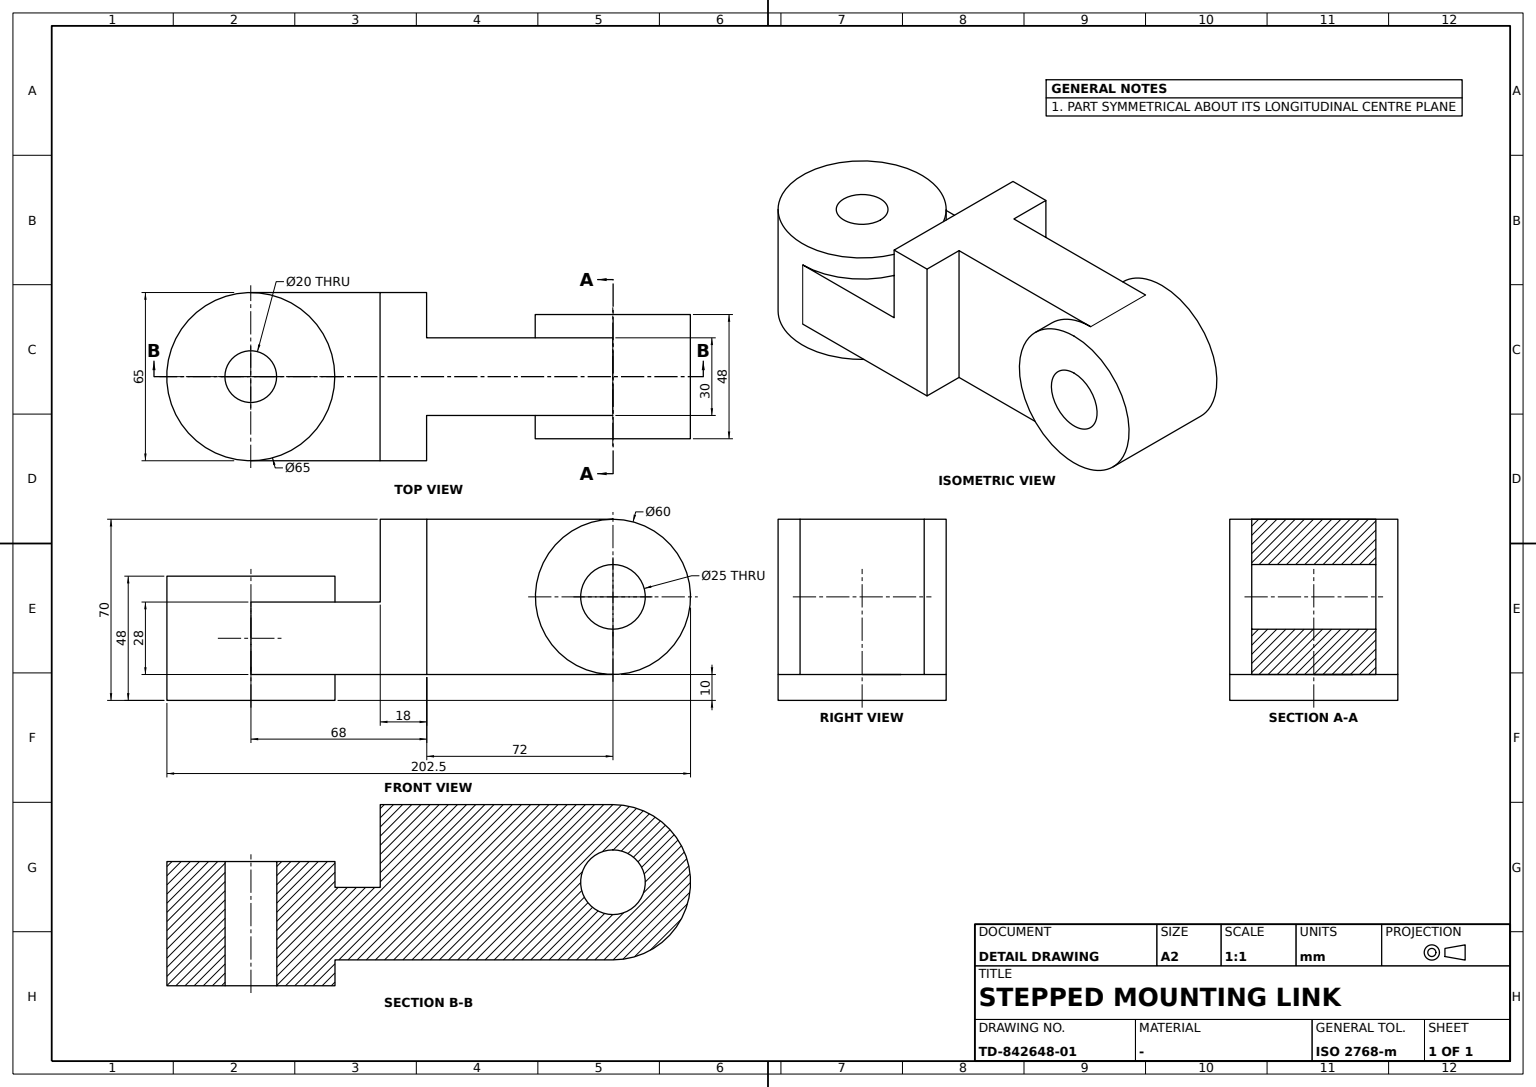
ISO-10303-21;
HEADER;
FILE_DESCRIPTION((''),'2;1');
FILE_NAME('','',(''),(''),'','','');
FILE_SCHEMA(('AUTOMOTIVE_DESIGN'));
ENDSEC;
DATA;
#1=APPLICATION_CONTEXT('');
#2=PRODUCT_CONTEXT('',#1,'mechanical');
#3=PRODUCT('','','',(#2));
#4=PRODUCT_DEFINITION_FORMATION('','',#3);
#5=PRODUCT_DEFINITION_CONTEXT('',#1,'design');
#6=PRODUCT_DEFINITION('','',#4,#5);
#7=PRODUCT_DEFINITION_SHAPE('','',#6);
#8=(LENGTH_UNIT()NAMED_UNIT(*)SI_UNIT(.MILLI.,.METRE.));
#9=(NAMED_UNIT(*)PLANE_ANGLE_UNIT()SI_UNIT($,.RADIAN.));
#10=(NAMED_UNIT(*)SI_UNIT($,.STERADIAN.)SOLID_ANGLE_UNIT());
#11=UNCERTAINTY_MEASURE_WITH_UNIT(LENGTH_MEASURE(0.005),#8,'distance_accuracy_value','');
#12=(GEOMETRIC_REPRESENTATION_CONTEXT(3)GLOBAL_UNCERTAINTY_ASSIGNED_CONTEXT((#11))GLOBAL_UNIT_ASSIGNED_CONTEXT((#8,#9,#10))REPRESENTATION_CONTEXT('',''));
#13=CARTESIAN_POINT('',(34.,-15.,0.));
#14=VERTEX_POINT('',#13);
#15=CARTESIAN_POINT('',(34.,-32.5,0.));
#16=VERTEX_POINT('',#15);
#17=CARTESIAN_POINT('',(34.,0.,0.));
#18=DIRECTION('',(0.,-1.,0.));
#19=VECTOR('',#18,1000.);
#20=LINE('',#17,#19);
#21=EDGE_CURVE('',#14,#16,#20,.T.);
#22=ORIENTED_EDGE('',*,*,#21,.F.);
#23=CARTESIAN_POINT('',(34.,-15.,60.));
#24=VERTEX_POINT('',#23);
#25=DIRECTION('',(0.,0.,-1.));
#26=VECTOR('',#25,1000.);
#27=LINE('',#13,#26);
#28=EDGE_CURVE('',#24,#14,#27,.T.);
#29=ORIENTED_EDGE('',*,*,#28,.F.);
#30=CARTESIAN_POINT('',(34.,-32.5,60.));
#31=VERTEX_POINT('',#30);
#32=CARTESIAN_POINT('',(34.,0.,60.));
#33=LINE('',#32,#19);
#34=EDGE_CURVE('',#24,#31,#33,.T.);
#35=ORIENTED_EDGE('',*,*,#34,.T.);
#36=DIRECTION('',(0.,0.,1.));
#37=VECTOR('',#36,1000.);
#38=LINE('',#15,#37);
#39=EDGE_CURVE('',#16,#31,#38,.T.);
#40=ORIENTED_EDGE('',*,*,#39,.F.);
#41=EDGE_LOOP('',(#22,#29,#35,#40));
#42=FACE_BOUND('',#41,.T.);
#43=CARTESIAN_POINT('',(34.,32.5,0.));
#44=DIRECTION('',(-1.,0.,0.));
#45=AXIS2_PLACEMENT_3D('',#43,#44,#18);
#46=PLANE('',#45);
#47=ADVANCED_FACE('',(#42),#46,.F.);
#48=CARTESIAN_POINT('',(-24.,0.,-10.));
#49=VERTEX_POINT('',#48);
#50=CARTESIAN_POINT('',(-34.,0.,-10.));
#51=DIRECTION('',(1.,0.,0.));
#52=AXIS2_PLACEMENT_3D('',#50,#36,#51);
#53=CIRCLE('',#52,10.);
#54=EDGE_CURVE('',#49,#49,#53,.T.);
#55=ORIENTED_EDGE('',*,*,#54,.F.);
#56=EDGE_LOOP('',(#55));
#57=FACE_BOUND('',#56,.T.);
#58=CARTESIAN_POINT('',(-24.,0.,38.));
#59=VERTEX_POINT('',#58);
#60=CARTESIAN_POINT('',(-34.,0.,38.));
#61=AXIS2_PLACEMENT_3D('',#60,#36,#51);
#62=CIRCLE('',#61,10.);
#63=EDGE_CURVE('',#59,#59,#62,.T.);
#64=ORIENTED_EDGE('',*,*,#63,.T.);
#65=EDGE_LOOP('',(#64));
#66=FACE_BOUND('',#65,.T.);
#67=CARTESIAN_POINT('',(-34.,0.,14.));
#68=AXIS2_PLACEMENT_3D('',#67,#36,#51);
#69=CYLINDRICAL_SURFACE('',#68,10.);
#70=ADVANCED_FACE('',(#57,#66),#69,.F.);
#71=ORIENTED_EDGE('',*,*,#54,.T.);
#72=EDGE_LOOP('',(#71));
#73=FACE_BOUND('',#72,.T.);
#74=CARTESIAN_POINT('',(-1.5,0.,-10.));
#75=VERTEX_POINT('',#74);
#76=CIRCLE('',#52,32.5);
#77=EDGE_CURVE('',#75,#75,#76,.T.);
#78=ORIENTED_EDGE('',*,*,#77,.F.);
#79=EDGE_LOOP('',(#78));
#80=FACE_BOUND('',#79,.T.);
#81=CARTESIAN_POINT('',(0.,0.,-10.));
#82=AXIS2_PLACEMENT_3D('',#81,#36,#51);
#83=PLANE('',#82);
#84=ADVANCED_FACE('',(#73,#80),#83,.F.);
#85=CARTESIAN_POINT('',(106.,-15.,0.));
#86=VERTEX_POINT('',#85);
#87=VECTOR('',#51,1000.);
#88=LINE('',#13,#87);
#89=EDGE_CURVE('',#14,#86,#88,.T.);
#90=ORIENTED_EDGE('',*,*,#89,.T.);
#91=CARTESIAN_POINT('',(106.,-15.,60.));
#92=VERTEX_POINT('',#91);
#93=CARTESIAN_POINT('',(106.,-15.,30.));
#94=DIRECTION('',(0.,1.,0.));
#95=AXIS2_PLACEMENT_3D('',#93,#94,#36);
#96=CIRCLE('',#95,30.);
#97=EDGE_CURVE('',#86,#92,#96,.T.);
#98=ORIENTED_EDGE('',*,*,#97,.T.);
#99=LINE('',#23,#87);
#100=EDGE_CURVE('',#24,#92,#99,.T.);
#101=ORIENTED_EDGE('',*,*,#100,.F.);
#102=ORIENTED_EDGE('',*,*,#28,.T.);
#103=EDGE_LOOP('',(#90,#98,#101,#102));
#104=FACE_BOUND('',#103,.T.);
#105=AXIS2_PLACEMENT_3D('',#23,#94,#51);
#106=PLANE('',#105);
#107=ADVANCED_FACE('',(#104),#106,.F.);
#108=CARTESIAN_POINT('',(16.,-32.5,28.));
#109=VERTEX_POINT('',#108);
#110=CARTESIAN_POINT('',(16.,-32.5,60.));
#111=VERTEX_POINT('',#110);
#112=CARTESIAN_POINT('',(16.,-32.5,0.));
#113=LINE('',#112,#37);
#114=EDGE_CURVE('',#109,#111,#113,.T.);
#115=ORIENTED_EDGE('',*,*,#114,.F.);
#116=CARTESIAN_POINT('',(-34.,-32.5,28.));
#117=VERTEX_POINT('',#116);
#118=CARTESIAN_POINT('',(0.,-32.5,28.));
#119=VECTOR('',#44,1000.);
#120=LINE('',#118,#119);
#121=EDGE_CURVE('',#109,#117,#120,.T.);
#122=ORIENTED_EDGE('',*,*,#121,.T.);
#123=CARTESIAN_POINT('',(-34.,-32.5,0.));
#124=VERTEX_POINT('',#123);
#125=CARTESIAN_POINT('',(-34.,-32.5,14.));
#126=LINE('',#125,#37);
#127=EDGE_CURVE('',#117,#124,#126,.F.);
#128=ORIENTED_EDGE('',*,*,#127,.T.);
#129=CARTESIAN_POINT('',(0.,-32.5,0.));
#130=LINE('',#129,#119);
#131=EDGE_CURVE('',#16,#124,#130,.T.);
#132=ORIENTED_EDGE('',*,*,#131,.F.);
#133=ORIENTED_EDGE('',*,*,#39,.T.);
#134=LINE('',#30,#87);
#135=EDGE_CURVE('',#111,#31,#134,.T.);
#136=ORIENTED_EDGE('',*,*,#135,.F.);
#137=EDGE_LOOP('',(#115,#122,#128,#132,#133,#136));
#138=FACE_BOUND('',#137,.T.);
#139=AXIS2_PLACEMENT_3D('',#15,#94,#44);
#140=PLANE('',#139);
#141=ADVANCED_FACE('',(#138),#140,.F.);
#142=CARTESIAN_POINT('',(106.,-24.,42.5));
#143=VERTEX_POINT('',#142);
#144=CARTESIAN_POINT('',(106.,-24.,30.));
#145=AXIS2_PLACEMENT_3D('',#144,#94,#36);
#146=CIRCLE('',#145,12.5);
#147=EDGE_CURVE('',#143,#143,#146,.F.);
#148=ORIENTED_EDGE('',*,*,#147,.F.);
#149=EDGE_LOOP('',(#148));
#150=FACE_BOUND('',#149,.T.);
#151=CARTESIAN_POINT('',(106.,-24.,60.));
#152=VERTEX_POINT('',#151);
#153=CIRCLE('',#145,30.);
#154=EDGE_CURVE('',#152,#152,#153,.T.);
#155=ORIENTED_EDGE('',*,*,#154,.F.);
#156=EDGE_LOOP('',(#155));
#157=FACE_BOUND('',#156,.T.);
#158=CARTESIAN_POINT('',(0.,-24.,0.));
#159=AXIS2_PLACEMENT_3D('',#158,#94,#44);
#160=PLANE('',#159);
#161=ADVANCED_FACE('',(#150,#157),#160,.F.);
#162=CARTESIAN_POINT('',(16.,32.5,28.));
#163=VERTEX_POINT('',#162);
#164=CARTESIAN_POINT('',(16.,32.5,60.));
#165=VERTEX_POINT('',#164);
#166=LINE('',#162,#37);
#167=EDGE_CURVE('',#163,#165,#166,.T.);
#168=ORIENTED_EDGE('',*,*,#167,.F.);
#169=CARTESIAN_POINT('',(16.,0.,28.));
#170=LINE('',#169,#19);
#171=EDGE_CURVE('',#163,#109,#170,.T.);
#172=ORIENTED_EDGE('',*,*,#171,.T.);
#173=ORIENTED_EDGE('',*,*,#114,.T.);
#174=CARTESIAN_POINT('',(16.,0.,60.));
#175=LINE('',#174,#19);
#176=EDGE_CURVE('',#165,#111,#175,.T.);
#177=ORIENTED_EDGE('',*,*,#176,.F.);
#178=EDGE_LOOP('',(#168,#172,#173,#177));
#179=FACE_BOUND('',#178,.T.);
#180=AXIS2_PLACEMENT_3D('',#162,#44,#18);
#181=PLANE('',#180);
#182=ADVANCED_FACE('',(#179),#181,.T.);
#183=CARTESIAN_POINT('',(-34.,32.5,0.));
#184=VERTEX_POINT('',#183);
#185=CARTESIAN_POINT('',(-34.,0.,0.));
#186=AXIS2_PLACEMENT_3D('',#185,#36,#51);
#187=CIRCLE('',#186,32.5);
#188=EDGE_CURVE('',#124,#184,#187,.T.);
#189=ORIENTED_EDGE('',*,*,#188,.F.);
#190=ORIENTED_EDGE('',*,*,#127,.F.);
#191=CARTESIAN_POINT('',(-34.,32.5,28.));
#192=VERTEX_POINT('',#191);
#193=CARTESIAN_POINT('',(-34.,0.,28.));
#194=AXIS2_PLACEMENT_3D('',#193,#36,#51);
#195=CIRCLE('',#194,32.5);
#196=EDGE_CURVE('',#117,#192,#195,.T.);
#197=ORIENTED_EDGE('',*,*,#196,.T.);
#198=CARTESIAN_POINT('',(-34.,32.5,14.));
#199=LINE('',#198,#37);
#200=EDGE_CURVE('',#192,#184,#199,.F.);
#201=ORIENTED_EDGE('',*,*,#200,.T.);
#202=EDGE_LOOP('',(#189,#190,#197,#201));
#203=FACE_BOUND('',#202,.T.);
#204=CARTESIAN_POINT('',(-1.5,0.,38.));
#205=VERTEX_POINT('',#204);
#206=CIRCLE('',#61,32.5);
#207=EDGE_CURVE('',#205,#205,#206,.T.);
#208=ORIENTED_EDGE('',*,*,#207,.F.);
#209=EDGE_LOOP('',(#208));
#210=FACE_BOUND('',#209,.T.);
#211=ORIENTED_EDGE('',*,*,#77,.T.);
#212=EDGE_LOOP('',(#211));
#213=FACE_BOUND('',#212,.T.);
#214=CYLINDRICAL_SURFACE('',#68,32.5);
#215=ADVANCED_FACE('',(#203,#210,#213),#214,.T.);
#216=ORIENTED_EDGE('',*,*,#171,.F.);
#217=CARTESIAN_POINT('',(0.,32.5,28.));
#218=LINE('',#217,#87);
#219=EDGE_CURVE('',#192,#163,#218,.T.);
#220=ORIENTED_EDGE('',*,*,#219,.F.);
#221=ORIENTED_EDGE('',*,*,#196,.F.);
#222=ORIENTED_EDGE('',*,*,#121,.F.);
#223=EDGE_LOOP('',(#216,#220,#221,#222));
#224=FACE_BOUND('',#223,.T.);
#225=CARTESIAN_POINT('',(0.,0.,28.));
#226=AXIS2_PLACEMENT_3D('',#225,#36,#51);
#227=PLANE('',#226);
#228=ADVANCED_FACE('',(#224),#227,.T.);
#229=ORIENTED_EDGE('',*,*,#63,.F.);
#230=EDGE_LOOP('',(#229));
#231=FACE_BOUND('',#230,.T.);
#232=ORIENTED_EDGE('',*,*,#207,.T.);
#233=EDGE_LOOP('',(#232));
#234=FACE_BOUND('',#233,.T.);
#235=CARTESIAN_POINT('',(0.,0.,38.));
#236=AXIS2_PLACEMENT_3D('',#235,#36,#51);
#237=PLANE('',#236);
#238=ADVANCED_FACE('',(#231,#234),#237,.T.);
#239=ORIENTED_EDGE('',*,*,#154,.T.);
#240=EDGE_LOOP('',(#239));
#241=FACE_BOUND('',#240,.T.);
#242=CARTESIAN_POINT('',(106.,15.,0.));
#243=VERTEX_POINT('',#242);
#244=CARTESIAN_POINT('',(106.,0.,0.));
#245=VECTOR('',#94,1000.);
#246=LINE('',#244,#245);
#247=EDGE_CURVE('',#86,#243,#246,.T.);
#248=ORIENTED_EDGE('',*,*,#247,.T.);
#249=CARTESIAN_POINT('',(106.,15.,60.));
#250=VERTEX_POINT('',#249);
#251=CARTESIAN_POINT('',(106.,15.,30.));
#252=AXIS2_PLACEMENT_3D('',#251,#18,#25);
#253=CIRCLE('',#252,30.);
#254=EDGE_CURVE('',#250,#243,#253,.T.);
#255=ORIENTED_EDGE('',*,*,#254,.F.);
#256=CARTESIAN_POINT('',(106.,0.,60.));
#257=LINE('',#256,#245);
#258=EDGE_CURVE('',#92,#250,#257,.T.);
#259=ORIENTED_EDGE('',*,*,#258,.F.);
#260=ORIENTED_EDGE('',*,*,#97,.F.);
#261=EDGE_LOOP('',(#248,#255,#259,#260));
#262=FACE_BOUND('',#261,.T.);
#263=CARTESIAN_POINT('',(106.,24.,60.));
#264=VERTEX_POINT('',#263);
#265=CARTESIAN_POINT('',(106.,24.,30.));
#266=AXIS2_PLACEMENT_3D('',#265,#94,#36);
#267=CIRCLE('',#266,30.);
#268=EDGE_CURVE('',#264,#264,#267,.T.);
#269=ORIENTED_EDGE('',*,*,#268,.F.);
#270=EDGE_LOOP('',(#269));
#271=FACE_BOUND('',#270,.T.);
#272=CARTESIAN_POINT('',(106.,0.,30.));
#273=AXIS2_PLACEMENT_3D('',#272,#94,#44);
#274=CYLINDRICAL_SURFACE('',#273,30.);
#275=ADVANCED_FACE('',(#241,#262,#271),#274,.T.);
#276=CARTESIAN_POINT('',(34.,15.,60.));
#277=VERTEX_POINT('',#276);
#278=LINE('',#249,#119);
#279=EDGE_CURVE('',#250,#277,#278,.T.);
#280=ORIENTED_EDGE('',*,*,#279,.F.);
#281=ORIENTED_EDGE('',*,*,#254,.T.);
#282=CARTESIAN_POINT('',(34.,15.,0.));
#283=VERTEX_POINT('',#282);
#284=LINE('',#242,#119);
#285=EDGE_CURVE('',#243,#283,#284,.T.);
#286=ORIENTED_EDGE('',*,*,#285,.T.);
#287=LINE('',#276,#26);
#288=EDGE_CURVE('',#277,#283,#287,.T.);
#289=ORIENTED_EDGE('',*,*,#288,.F.);
#290=EDGE_LOOP('',(#280,#281,#286,#289));
#291=FACE_BOUND('',#290,.T.);
#292=AXIS2_PLACEMENT_3D('',#249,#18,#44);
#293=PLANE('',#292);
#294=ADVANCED_FACE('',(#291),#293,.F.);
#295=ORIENTED_EDGE('',*,*,#268,.T.);
#296=EDGE_LOOP('',(#295));
#297=FACE_BOUND('',#296,.T.);
#298=CARTESIAN_POINT('',(106.,24.,42.5));
#299=VERTEX_POINT('',#298);
#300=CIRCLE('',#266,12.5);
#301=EDGE_CURVE('',#299,#299,#300,.F.);
#302=ORIENTED_EDGE('',*,*,#301,.T.);
#303=EDGE_LOOP('',(#302));
#304=FACE_BOUND('',#303,.T.);
#305=CARTESIAN_POINT('',(0.,24.,0.));
#306=AXIS2_PLACEMENT_3D('',#305,#94,#44);
#307=PLANE('',#306);
#308=ADVANCED_FACE('',(#297,#304),#307,.T.);
#309=CARTESIAN_POINT('',(34.,32.5,60.));
#310=VERTEX_POINT('',#309);
#311=CARTESIAN_POINT('',(-34.,32.5,60.));
#312=LINE('',#311,#119);
#313=EDGE_CURVE('',#310,#165,#312,.T.);
#314=ORIENTED_EDGE('',*,*,#313,.F.);
#315=VERTEX_POINT('',#43);
#316=LINE('',#43,#37);
#317=EDGE_CURVE('',#315,#310,#316,.T.);
#318=ORIENTED_EDGE('',*,*,#317,.F.);
#319=CARTESIAN_POINT('',(0.,32.5,0.));
#320=LINE('',#319,#87);
#321=EDGE_CURVE('',#184,#315,#320,.T.);
#322=ORIENTED_EDGE('',*,*,#321,.F.);
#323=ORIENTED_EDGE('',*,*,#200,.F.);
#324=ORIENTED_EDGE('',*,*,#219,.T.);
#325=ORIENTED_EDGE('',*,*,#167,.T.);
#326=EDGE_LOOP('',(#314,#318,#322,#323,#324,#325));
#327=FACE_BOUND('',#326,.T.);
#328=AXIS2_PLACEMENT_3D('',#183,#18,#51);
#329=PLANE('',#328);
#330=ADVANCED_FACE('',(#327),#329,.F.);
#331=ORIENTED_EDGE('',*,*,#147,.T.);
#332=EDGE_LOOP('',(#331));
#333=FACE_BOUND('',#332,.T.);
#334=ORIENTED_EDGE('',*,*,#301,.F.);
#335=EDGE_LOOP('',(#334));
#336=FACE_BOUND('',#335,.T.);
#337=AXIS2_PLACEMENT_3D('',#272,#18,#51);
#338=CYLINDRICAL_SURFACE('',#337,12.5);
#339=ADVANCED_FACE('',(#333,#336),#338,.F.);
#340=ORIENTED_EDGE('',*,*,#131,.T.);
#341=ORIENTED_EDGE('',*,*,#188,.T.);
#342=ORIENTED_EDGE('',*,*,#321,.T.);
#343=EDGE_CURVE('',#315,#283,#20,.T.);
#344=ORIENTED_EDGE('',*,*,#343,.T.);
#345=ORIENTED_EDGE('',*,*,#285,.F.);
#346=ORIENTED_EDGE('',*,*,#247,.F.);
#347=ORIENTED_EDGE('',*,*,#89,.F.);
#348=ORIENTED_EDGE('',*,*,#21,.T.);
#349=EDGE_LOOP('',(#340,#341,#342,#344,#345,#346,#347,#348));
#350=FACE_BOUND('',#349,.T.);
#351=CARTESIAN_POINT('',(0.,0.,0.));
#352=AXIS2_PLACEMENT_3D('',#351,#36,#51);
#353=PLANE('',#352);
#354=ADVANCED_FACE('',(#350),#353,.F.);
#355=ORIENTED_EDGE('',*,*,#288,.T.);
#356=ORIENTED_EDGE('',*,*,#343,.F.);
#357=ORIENTED_EDGE('',*,*,#317,.T.);
#358=EDGE_CURVE('',#310,#277,#33,.T.);
#359=ORIENTED_EDGE('',*,*,#358,.T.);
#360=EDGE_LOOP('',(#355,#356,#357,#359));
#361=FACE_BOUND('',#360,.T.);
#362=ADVANCED_FACE('',(#361),#46,.F.);
#363=ORIENTED_EDGE('',*,*,#358,.F.);
#364=ORIENTED_EDGE('',*,*,#313,.T.);
#365=ORIENTED_EDGE('',*,*,#176,.T.);
#366=ORIENTED_EDGE('',*,*,#135,.T.);
#367=ORIENTED_EDGE('',*,*,#34,.F.);
#368=ORIENTED_EDGE('',*,*,#100,.T.);
#369=ORIENTED_EDGE('',*,*,#258,.T.);
#370=ORIENTED_EDGE('',*,*,#279,.T.);
#371=EDGE_LOOP('',(#363,#364,#365,#366,#367,#368,#369,#370));
#372=FACE_BOUND('',#371,.T.);
#373=CARTESIAN_POINT('',(0.,0.,60.));
#374=AXIS2_PLACEMENT_3D('',#373,#36,#51);
#375=PLANE('',#374);
#376=ADVANCED_FACE('',(#372),#375,.T.);
#377=CLOSED_SHELL('',(#47,#70,#84,#107,#141,#161,#182,#215,#228,#238,#275,#294,#308,#330,#339,#354,#362,#376));
#378=MANIFOLD_SOLID_BREP('',#377);
#379=ADVANCED_BREP_SHAPE_REPRESENTATION('',(#378),#12);
#380=SHAPE_DEFINITION_REPRESENTATION(#7,#379);
ENDSEC;
END-ISO-10303-21;
